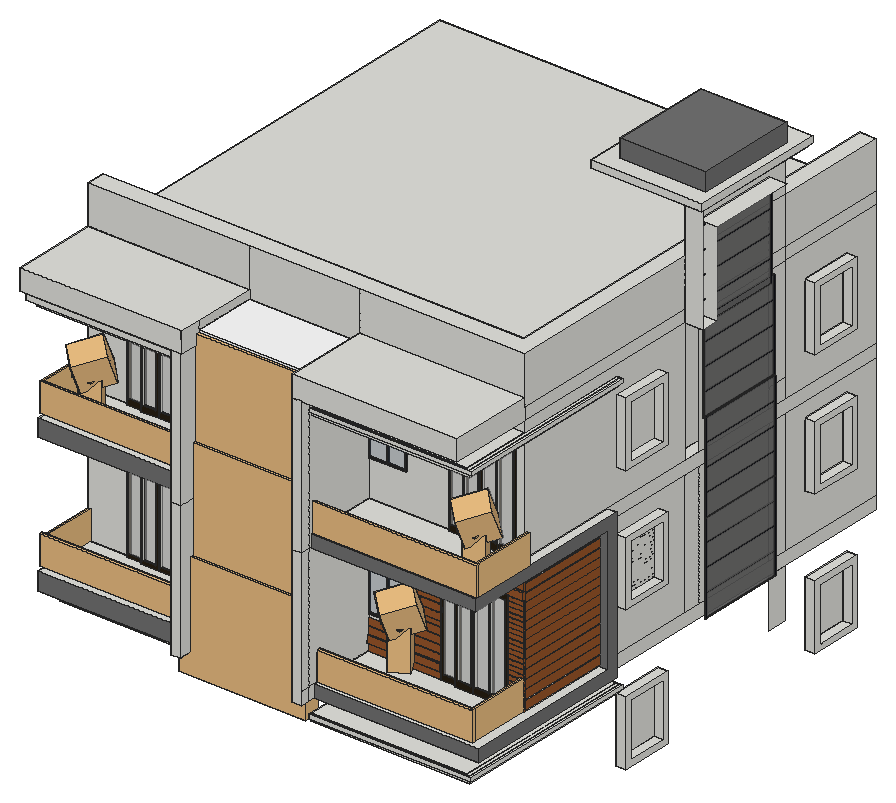
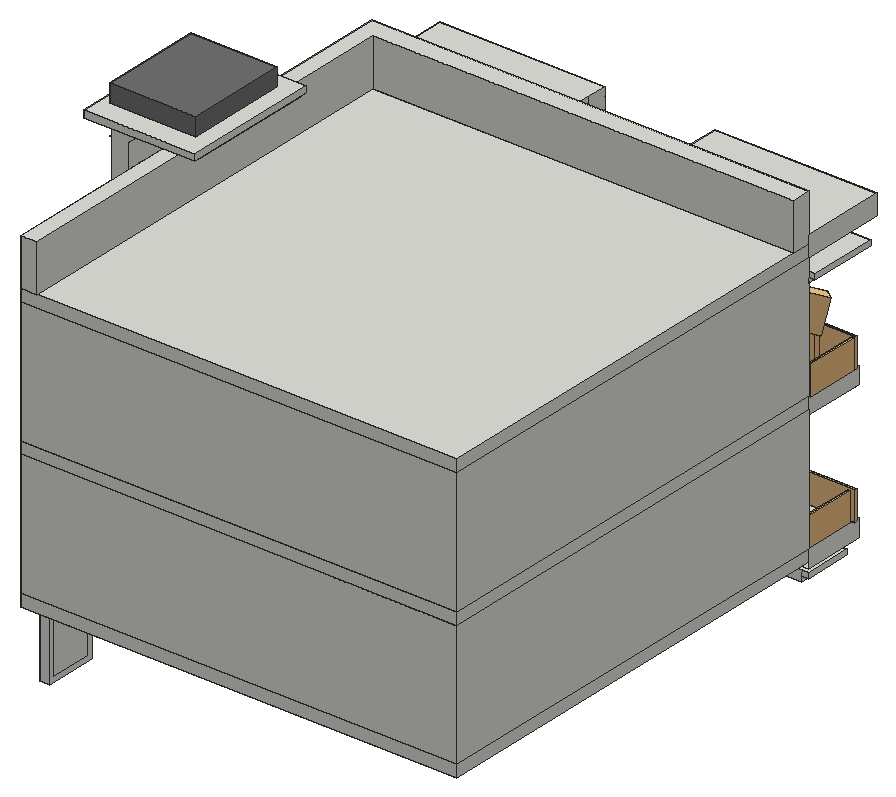
# SketchUp Ruby script. Lengths in inches.
U = 1.inch
M = Sketchup.active_model
def pt(a) = Geom::Point3d.new(a.map { |v| v * U })
def face(e, loops, mat)
  f = e.add_face(loops[0].map { |a| pt(a) })
  loops[1..].each { |l| e.add_face(l.map { |a| pt(a) }).erase! }
  f.material = f.back_material = mat if mat
  f
end
# faces: each face lists its corners as indices into pts; further lists are holes
def faces(e, pts, list, mat = nil) = list.each { |f| face(e, (f[0].is_a?(Array) ? f : [f]).map { |l| l.map { |i| pts[i] } }, mat) }
# xy, xz, yz: faces in a plane at the given z, y or x. An outline is a flat list of corners, or four numbers for a rectangle; further outlines are holes
def ring(l) = l.size == 4 ? [[l[0], l[1]], [l[2], l[1]], [l[2], l[3]], [l[0], l[3]]] : l.each_slice(2).to_a
def flat(e, list, mat, &to3) = list.each { |f| face(e, (f[0].is_a?(Array) ? f : [f]).map { |l| ring(l).map { |u, v| to3.(u, v) } }, mat) }
def xy(e, z, list, mat = nil) = flat(e, list, mat) { |x, y| [x, y, z] }
def xz(e, y, list, mat = nil) = flat(e, list, mat) { |x, z| [x, y, z] }
def yz(e, x, list, mat = nil) = flat(e, list, mat) { |y, z| [x, y, z] }
def lines(e, pts, list) = list.each { |a, b| e.add_line(pt(pts[a]), pt(pts[b])) }
# prism: a flat outline (further loops are holes) pulled along v
def prism(e, loops, v, mat = nil)
  f = face(e, loops, mat); d = Geom::Vector3d.new(v.map { |x| x * U })
  f.pushpull(f.normal.samedirection?(d) ? d.length : -d.length)
end
def box(e, o, s, mat = nil) = prism(e, [[o, [o[0] + s[0], o[1], o[2]], [o[0] + s[0], o[1] + s[1], o[2]], [o[0], o[1] + s[1], o[2]]]], [0, 0, s[2]], mat)
def at(x, y, z, deg = 0) = Geom::Transformation.translation(pt([x, y, z])) * Geom::Transformation.rotation(ORIGIN, Z_AXIS, deg.degrees)
def axes(o, x, y, z) = Geom::Transformation.new([*x, 0, *y, 0, *z, 0, *pt(o).to_a, 1])
def part(name) = M.definitions.add(name)
# library, detail: a bought-in or finely detailed component or shape, given as its bounding box
def library(name, o, s) = part(name).tap { |d| box(d.entities, o, s) }
def detail(e, o, s) = box(e.add_group.entities, o, s)
def put(e, d, t, mat = nil) = e.add_instance(d, t).tap { |i| i.material = mat if mat }
def group(e, t, mat = nil) = e.add_group.tap { |g| g.transformation = t; g.material = mat if mat }.entities
root = M.entities
M.materials.add("Material__1").color = [51, 42, 44]
M.materials.add("Material__2").color = [97, 132, 37]
M.materials.add("[0136_Charcoal]").color = [35, 35, 35]
M.materials.add("[Color M00]").color = [255, 255, 255]
M.materials.add("[Color M05]").color = [114, 114, 114]
M.materials.add("[Translucent Glass Gray]2").color = [201, 201, 201]
M.materials["[Translucent Glass Gray]2"].alpha = 0.5
M.materials.add("[Translucent_Glass_Blue]").color = [68, 104, 165]
M.materials["[Translucent_Glass_Blue]"].alpha = 0.07
M.materials.add("[Translucent_Glass_Green_Dark]").color = [33, 68, 103]
M.materials["[Translucent_Glass_Green_Dark]"].alpha = 0.08
M.materials.add("[Wood Cherry Original]").color = [152, 86, 42]
M.materials.add("oak swatch").color = [40, 31, 19]
M.materials.add("{045efeae-c101-a24d-bd9b-6f5600100adb}").color = [102, 102, 102]
M.materials["{045efeae-c101-a24d-bd9b-6f5600100adb}"].alpha = 0.7
M.materials.add("{16756a1b-d383-d94f-ad82-104813d2624f}").color = [19, 21, 27]
c1 = part("Group\#20")
xy(c1.entities,0,[[[0,0,50.8125,62.9375],[5.49,5.49,45.32,57.45]],[5.49,5.49,45.32,57.45]])
xy(c1.entities,9.5625,[[[0,0,50.8125,62.9375],[5.49,5.49,45.32,57.45]]])
xz(c1.entities,0,[[0,0,50.8125,9.5625]])
xz(c1.entities,5.49,[[5.49,0,45.32,9.5625]])
xz(c1.entities,57.45,[[5.49,0,45.32,9.5625]])
xz(c1.entities,62.9375,[[0,0,50.8125,9.5625]])
yz(c1.entities,0,[[0,0,62.9375,9.5625]])
yz(c1.entities,5.49,[[5.49,0,57.45,9.5625]])
yz(c1.entities,45.32,[[5.49,0,57.45,9.5625]])
yz(c1.entities,50.8125,[[0,0,62.9375,9.5625]])
c2 = library("Facade Louver",[-2.17,-1,-2.17],[122.45,14.39,102.76])
c3 = part("Group\#29")
xy(c3.entities,-4.5625,[[0,-81.875,145.875,0]])
xy(c3.entities,0.59,[[-6.375,-89.375,-6.375,0,0,0,0,-81.875,145.875,-81.875,145.875,-89.375]])
xy(c3.entities,5.73,[[-6.375,-89.375,145.875,0]])
xz(c3.entities,-89.375,[[-6.375,0.59,145.875,5.73]])
xz(c3.entities,-81.875,[[0,-4.5625,145.875,0.59]])
xz(c3.entities,0,[[0,-4.5625,145.875,5.73],[-6.375,0.59,0,5.73]])
yz(c3.entities,-6.375,[[-89.375,0.59,0,5.73]])
yz(c3.entities,0,[[-81.875,-4.5625,0,0.59]])
yz(c3.entities,145.875,[[-81.875,-4.5625,0,-4.5625,0,5.73,-89.375,5.73,-89.375,0.59,-81.875,0.59]])
c4 = part("Furniture_0DcpanrIvuI8n_9Ae92L5A")
g1 = group(c4.entities,at(0,0,0))
box(g1,[-19.29,-0.2,0.39],[38.58,0.4,83.86],"{045efeae-c101-a24d-bd9b-6f5600100adb}")
g2 = group(c4.entities,at(0,0,0))
box(g2,[-19.68,-0.59,63.39],[39.36,1.18,0.39],"{16756a1b-d383-d94f-ad82-104813d2624f}")
box(g2,[-19.68,-0.59,42.52],[39.36,1.18,0.39],"{16756a1b-d383-d94f-ad82-104813d2624f}")
box(g2,[-19.68,-0.59,21.26],[39.36,1.18,0.39],"{16756a1b-d383-d94f-ad82-104813d2624f}")
xy(g2,0,[[-19.68,-0.59,19.68,0.59]],"{16756a1b-d383-d94f-ad82-104813d2624f}")
xy(g2,0.39,[[-19.68,-0.59,-19.29,0.59],[-19.68,-0.59,19.68,0.59],[19.29,-0.59,19.68,0.59]],"{16756a1b-d383-d94f-ad82-104813d2624f}")
xy(g2,84.25,[[-19.68,-0.59,19.68,0.59]],"{16756a1b-d383-d94f-ad82-104813d2624f}")
xy(g2,84.65,[[-19.68,-0.59,-19.29,0.59],[-19.68,-0.59,19.68,0.59],[19.29,-0.59,19.68,0.59]],"{16756a1b-d383-d94f-ad82-104813d2624f}")
xz(g2,-0.59,[[-19.68,0,19.68,0.39],[-19.68,0.39,-19.29,84.65],[19.29,0.39,19.68,84.65],[-19.68,84.25,19.68,84.65]],"{16756a1b-d383-d94f-ad82-104813d2624f}")
xz(g2,0.59,[[-19.68,0,19.68,0.39],[-19.68,0.39,-19.29,84.65],[19.29,0.39,19.68,84.65],[-19.68,84.25,19.68,84.65]],"{16756a1b-d383-d94f-ad82-104813d2624f}")
yz(g2,-19.68,[[-0.59,0,0.59,0.39],[-0.59,0.39,0.59,84.65],[-0.59,84.25,0.59,84.65]],"{16756a1b-d383-d94f-ad82-104813d2624f}")
yz(g2,-19.29,[[-0.59,0.39,0.59,84.65]],"{16756a1b-d383-d94f-ad82-104813d2624f}")
yz(g2,19.29,[[-0.59,0.39,0.59,84.65]],"{16756a1b-d383-d94f-ad82-104813d2624f}")
yz(g2,19.68,[[-0.59,0,0.59,0.39],[-0.59,0.39,0.59,84.65],[-0.59,84.25,0.59,84.65]],"{16756a1b-d383-d94f-ad82-104813d2624f}")
c5 = part("Glass Window")
put(c5.entities,c4,at(0,0,-42.32))
c6 = part("Group\#7")
box(c6.entities,[0,0,0],[1.77,4.72,80.31],"oak swatch")
c7 = part("Exterior Sliding Doors")
xy(c7.entities,0,[[1.77,33.07,3.54,70.87],[1.77,70.87,3.54,108.66]])
xy(c7.entities,0,[[0,0,1.77,33.07],[0,108.66,1.77,141.73]],"oak swatch")
xy(c7.entities,4.72,[[0,4.72,1.77,33.07],[1.77,37.8,3.54,66.14],[1.77,75.88,3.54,103.9375],[0,108.66,1.77,137.01]],"oak swatch")
xy(c7.entities,75.59,[[1.77,37.8,3.54,66.14],[1.77,75.88,3.54,103.9375]])
xy(c7.entities,75.59,[[0,4.72,1.77,33.07],[0,108.66,1.77,137.01]],"oak swatch")
xy(c7.entities,80.31,[[0,0,1.77,33.07],[1.77,33.07,3.54,70.87],[1.77,70.87,3.54,108.66],[0,108.66,1.77,141.73]],"oak swatch")
xz(c7.entities,0,[[0,0,1.77,80.31]],"oak swatch")
xz(c7.entities,4.72,[[0,4.72,1.77,75.59]],"oak swatch")
xz(c7.entities,33.07,[[0,0,1.77,4.72],[1.77,0,3.54,80.31],[0,75.59,1.77,80.31]],"oak swatch")
xz(c7.entities,37.8,[[1.77,4.72,3.54,75.59]])
xz(c7.entities,66.14,[[1.77,4.72,3.54,75.59]],"oak swatch")
xz(c7.entities,70.87,[[1.77,0,3.54,80.31]])
xz(c7.entities,75.88,[[1.77,4.72,3.54,75.59]])
xz(c7.entities,103.9375,[[1.77,4.72,3.54,75.59]],"oak swatch")
xz(c7.entities,108.66,[[1.77,4.72,3.54,75.59]])
xz(c7.entities,108.66,[[0,0,3.54,4.72],[0,75.59,3.54,80.31]],"oak swatch")
xz(c7.entities,137.01,[[0,4.72,1.77,75.59]],"oak swatch")
xz(c7.entities,141.73,[[0,0,1.77,80.31]],"oak swatch")
yz(c7.entities,0,[[0,0,33.07,0,33.07,4.72,4.72,4.72,4.72,75.59,33.07,75.59,33.07,80.31,0,80.31],[108.66,0,141.73,0,141.73,80.31,108.66,80.31,108.66,75.59,137.01,75.59,137.01,4.72,108.66,4.72]],"oak swatch")
yz(c7.entities,1.77,[[4.72,4.72,33.07,75.59],[37.8,4.72,66.14,75.59],[75.88,4.72,103.9375,75.59],[108.66,4.72,137.01,75.59]],"[Translucent Glass Gray]2")
yz(c7.entities,1.77,[[0,0,33.07,0,33.07,4.72,4.72,4.72,4.72,75.59,33.07,75.59,33.07,80.31,0,80.31],[[33.07,0,70.87,80.31],[37.8,4.72,66.14,75.59]],[[70.87,0,141.73,80.31],[108.66,4.72,137.01,75.59],[75.88,4.72,103.9375,75.59]]],"oak swatch")
yz(c7.entities,3.54,[[[33.07,0,70.87,80.31],[37.8,4.72,66.14,75.59]],[[70.87,0,108.66,80.31],[75.88,4.72,103.9375,75.59]]],"oak swatch")
put(c7.entities,c6,at(0,33.07,0))
put(c7.entities,c6,at(0,103.9375,0))
c8 = part("Group\#15")
box(c8.entities,[0,0,0],[15.2,4.13,1.25])
c9 = library("Glass Railings(black Handrails)",[-57.04,-132.55,0],[169.29,2.52,28.17])
c10 = part("Group\#13")
box(c10.entities,[0,-0.9375,0],[71.3,0.9375,6.72])
c11 = part("Group\#8")
box(c11.entities,[61.69,-1.625,-2],[88.94,1.625,7.49])
c12 = library("\#1",[-138.85,-135.75,0],[277.7,270.97,9.64])
c13 = library("\#2",[-34.84,-73.35,-33.91],[69.68,146.26,68.31])
c14 = library("\#5",[-4127.85,-1300.75,-2324.72],[5349.84,4521.24,5423.31])
c15 = part("\#3")
put(c15.entities,c14,at(450.18,-1111.4375,0),"Material__2")
c16 = part("12")
put(c16.entities,c12,axes([-49.79,-36.9375,349.64],[0.59279,0,0],[0,0.59279,0],[0,0,0.59279]),"Material__1")
put(c16.entities,c13,axes([-39.24,-18.18,177.19],[1.20819,-2.09264,0],[0,0,2.41638],[2.09264,1.20819,0]))
put(c16.entities,c15,axes([-83.44,-46.04,442.44],[-0.03636,-0.03293,-0.01473],[-0.00083,-0.02391,0.05549],[0.02997,-0.02791,-0.01158]))
c17 = part("Group\#14")
box(c17.entities,[0,0,0],[34.99,6.92,0.9375])
c18 = part("Two-panel window \#1")
xy(c18.entities,-18,[[0,-31,2,35]],"[0136_Charcoal]")
xy(c18.entities,-16,[[0,-29,0.9375,33],[0.9375,-29,1.125,33],[1.125,-29,2,1],[1.125,3,2,33]],"[0136_Charcoal]")
xy(c18.entities,76,[[0,-29,0.9375,33],[0.9375,-29,1.125,33],[1.125,-29,2,1],[1.125,3,2,33]],"[0136_Charcoal]")
xy(c18.entities,78,[[0,-31,2,35]],"[0136_Charcoal]")
xz(c18.entities,-31,[[0,-18,2,78]],"[0136_Charcoal]")
xz(c18.entities,-29,[[0,-16,0.9375,76],[0.9375,-16,1.125,76],[1.125,-16,2,76]],"[0136_Charcoal]")
xz(c18.entities,1,[[1.125,-16,2,76]],"[0136_Charcoal]")
xz(c18.entities,3,[[1.125,-16,2,76]],"[0136_Charcoal]")
xz(c18.entities,33,[[0,-16,0.9375,76],[0.9375,-16,1.125,76],[1.125,-16,2,76]],"[0136_Charcoal]")
xz(c18.entities,35,[[0,-18,2,78]],"[0136_Charcoal]")
yz(c18.entities,0,[[[-31,-18,35,78],[-29,-16,33,76]]],"[0136_Charcoal]")
yz(c18.entities,0.9375,[[-29,-16,33,76]],"[Translucent_Glass_Blue]")
yz(c18.entities,1.125,[[1,-16,3,76]],"[0136_Charcoal]")
yz(c18.entities,1.125,[[-29,-16,1,76],[3,-16,33,76]],"[Translucent_Glass_Green_Dark]")
yz(c18.entities,2,[[[-31,-18,35,78],[-29,-16,1,76],[3,-16,33,76]]],"[0136_Charcoal]")
c19 = part("Two-panel window")
put(c19.entities,c18,axes([-31.84,50.72,0],[1,0,0],[0,1.1,0],[0,0,1]))
c20 = part("normal window")
put(c20.entities,c19,axes([114.26,44.3125,18],[0,1,0],[-0.90909,0,0],[0,0,1]))
prism(root,[[[317.76,103.01,369.07],[468.38,103.01,369.07],[468.38,173.57,369.07],[468.38,283.99,369.07],[474.57,283.99,369.07],[474.57,100.51,369.07],[317.76,100.51,369.07],[317.76,100.69,369.07]]],[0,0,3.5])
xy(root,378.5,[[45.88,113.44,191.76,173.57]])
xy(root,384,[[317.76,107.01,317.76,173.57,468.38,173.57,468.38,273.38,477.41,273.38,477.41,107.01]])
xy(root,396,[[317.76,107.01,477.41,107.01,477.41,262.5,468.38,262.5,468.38,173.57,317.76,173.57],[200.76,112.2,308.76,121.2],[45.88,113.44,191.76,173.57],[200.76,121.2,308.76,121.2,308.76,182.57,425.76,182.57,425.76,442.69,83.76,442.69,83.76,182.57,200.76,182.57],[45.88,173.57,200.76,173.57,200.76,182.57,83.76,182.57,83.76,442.69,425.76,442.69,425.76,182.57,308.76,182.57,308.76,173.57,468.38,173.57,468.38,598.82,45.88,598.82]])
xy(root,500.875,[[202.09,121.2,202.09,173.57,200.76,173.57,200.76,182.57,56.45,182.57,56.45,442.69,456.2,442.69,456.2,182.57,308.76,182.57,308.76,121.2]])
xy(root,511.75,[[45.88,113.44,191.76,173.57]])
xy(root,516,[[308.76,91.69,317.76,173.57],[200.76,112.2,308.76,121.2],[317.76,113.44,468.38,173.57],[45.88,173.57,200.76,173.57,200.76,182.57,83.76,182.57,83.76,442.69,425.76,442.69,425.76,182.57,308.76,182.57,308.76,173.57,468.38,173.57,468.38,598.82,45.88,598.82]])
xy(root,516.15,[[317.76,102.75,317.76,113.44,468.38,113.44,468.38,262.5,477.41,262.5,477.41,102.75]])
xy(root,528,[[317.76,102.75,477.41,102.75,477.41,273.38,468.38,273.38,468.38,113.44,317.76,113.44],[200.76,112.2,308.76,121.2],[45.88,113.44,191.76,173.57],[317.76,113.44,468.38,173.57],[200.76,121.2,308.76,121.2,308.76,182.57,456.2,182.57,456.2,442.69,56.45,442.69,56.45,182.57,200.76,182.57],
  [45.88,173.57,200.76,173.57,200.76,182.57,56.45,182.57,56.45,442.69,456.2,442.69,456.2,182.57,308.76,182.57,308.76,173.57,468.38,173.57,468.38,598.82,45.88,598.82]])
xy(root,634.26,[[317.76,101.26,317.76,103.01,468.38,103.01,468.38,284.44,475.01,284.44,475.01,101.26]])
xy(root,637.76,[[317.76,101.26,475.01,101.26,475.01,284.44,468.38,284.44,468.38,103.01,317.76,103.01]])
xy(root,648,[[45.88,91.69,83.76,173.57],[83.76,91.69,191.76,173.57],[191.76,91.69,200.76,173.57],[200.76,91.69,202.09,112.2],[308.76,91.69,317.76,173.57],
  [317.76,91.69,425.76,173.57],[425.76,91.69,468.38,173.57],[200.76,112.2,202.09,121.2],[202.09,112.2,308.76,121.2],[200.76,121.2,202.09,173.57],
  [45.88,173.57,200.76,173.57,200.76,182.57,56.45,182.57,56.45,442.69,456.2,442.69,456.2,182.57,308.76,182.57,308.76,173.57,468.38,173.57,468.38,598.82,45.88,598.82],[468.38,367.14,485.45,384.58]])
xy(root,660,[[45.88,173.57,45.88,192.04,452.39,192.04,452.39,598.82,468.38,598.82,468.38,173.57]])
xy(root,660,[[202.09,112.2,308.76,173.57]],"[Color M00]")
xy(root,668.0625,[[45.88,91.69,202.09,173.57],[308.76,91.69,468.38,173.57]])
xy(root,705.6875,[[45.88,173.57,468.38,173.57,468.38,598.82,452.39,598.82,452.39,192.04,45.88,192.04]])
xy(root,729.3125,[[468.38,384.58,485.45,469.33]])
xy(root,754.625,[[382.24,360.76,485.45,367.14],[485.45,360.76,489.76,488.7],[382.24,367.14,468.38,488.7],[468.38,367.14,485.45,488.7],[382.24,488.7,489.76,495.14]])
xy(root,761.4375,[[[382.24,360.76,489.76,495.14],[398.09,376.66,481.09,474.6]]])
xy(root,778.875,[[398.09,376.66,481.09,474.6]],"[Color M05]")
xz(root,91.69,[[191.76,383.9375,200.76,384],[191.76,384,200.76,516],[308.76,384,317.76,516],[191.76,516,200.76,648],[308.76,516,317.76,648],
  [45.88,648,202.09,668.0625],[308.76,648,468.38,668.0625]])
xz(root,101.26,[[317.76,634.26,475.01,637.76]])
xz(root,102.75,[[317.76,516.15,477.41,528]],"[Color M05]")
xz(root,103.01,[[317.76,634.26,468.38,637.76]])
xz(root,107.01,[[317.76,384,477.41,396]],"[Color M05]")
xz(root,112.2,[[200.76,384,308.76,396],[200.76,396,308.76,516],[200.76,516,308.76,528],[200.76,528,308.76,648]])
xz(root,112.2,[[202.09,648,308.76,660]],"[Color M00]")
xz(root,113.44,[[317.76,516,468.38,516.15],[317.76,516.15,468.38,528]])
xz(root,113.44,[[45.88,378.5,191.76,396],[45.88,511.75,191.76,528]],"[Color M05]")
xz(root,121.2,[[200.76,396,200.76,516,202.09,516,202.09,500.875,308.76,500.875,308.76,396],[202.09,500.875,308.76,516],[202.09,516,308.76,528],[200.76,528,202.09,648],[202.09,528,308.76,648]])
xz(root,173.57,[[191.76,383.9375,200.76,396],[308.76,384,317.76,396],[45.88,396,191.76,511.75],[389.06,396,468.38,396,468.38,508.52,317.76,508.52,317.76,402.72,389.06,402.72],[200.76,500.875,202.09,648],
  [45.88,511.75,191.76,516],[191.76,516,200.76,528],[308.76,516,317.76,528],[317.76,516,468.38,528],[45.88,528,191.76,630.49],
  [317.76,528,468.38,648],[45.88,641.6,191.76,648],[45.88,648,202.09,660],[308.76,648,468.38,660],[45.88,660,202.09,668.0625],
  [202.09,660,308.76,705.6875],[308.76,660,468.38,668.0625],[45.88,668.0625,202.09,705.6875],[308.76,668.0625,468.38,705.6875]])
xz(root,182.57,[[83.76,396,200.76,500.875],[308.76,396,425.76,500.875],[56.45,500.875,83.76,500.875,83.76,516,200.76,516,200.76,528,56.45,528],[83.76,500.875,200.76,516],[308.76,500.875,425.76,516],
  [425.76,500.875,456.2,500.875,456.2,528,308.76,528,308.76,516,425.76,516],[56.45,528,200.76,648],[308.76,528,456.2,648]])
xz(root,192.04,[[45.88,660,452.39,705.6875]])
xz(root,262.5,[[468.38,396,477.41,516.15]],"[Color M05]")
xz(root,273.38,[[468.38,384,477.41,528]])
xz(root,284.44,[[468.38,634.26,475.01,637.76]])
xz(root,360.76,[[382.24,754.625,489.76,761.4375]])
xz(root,367.14,[[468.38,648,485.45,754.625]])
xz(root,376.66,[[398.09,761.4375,481.09,778.875]],"[Color M05]")
xz(root,384.58,[[468.38,648,485.45,729.3125]])
xz(root,442.69,[[83.76,396,425.76,500.875],[56.45,500.875,56.45,528,456.2,528,456.2,500.875,425.76,500.875,425.76,516,83.76,516,83.76,500.875],[83.76,500.875,425.76,516],[56.45,528,456.2,648]])
xz(root,474.6,[[398.09,761.4375,481.09,778.875]],"[Color M05]")
xz(root,495.14,[[382.24,754.625,489.76,761.4375]])
xz(root,598.82,[[45.88,396,468.38,516],[45.88,528,468.38,648],[452.39,660,468.38,705.6875]])
yz(root,45.88,[[113.44,378.5,173.57,396],[173.57,396,598.82,516],[113.44,511.75,173.57,528],[173.57,528,598.82,648],[91.69,648,173.57,668.0625],
  [173.57,660,192.04,705.6875]])
yz(root,56.45,[[182.57,500.875,442.69,528],[182.57,528,442.69,648]])
yz(root,83.76,[[182.57,396,442.69,516]])
yz(root,191.76,[[113.44,378.5,173.57,396],[91.69,383.9375,100.69,384],[91.69,384,100.69,516],[113.44,511.75,173.57,528],[91.69,516,91.69,648,100.69,648,100.69,528,113.44,528,113.44,516],
  [100.69,528,173.57,648]])
yz(root,200.76,[[91.69,383.9375,112.2,384],[112.2,383.9375,121.2,396],[121.2,383.9375,173.57,384],[91.69,384,112.2,516],[121.2,384,173.57,396],
  [112.2,396,121.2,516],[121.2,396,182.57,396,182.57,500.875,173.57,500.875,173.57,516,121.2,516],[173.57,500.875,182.57,516],[91.69,516,112.2,648],[112.2,516,121.2,528],
  [121.2,516,173.57,528],[173.57,516,182.57,528],[121.2,528,173.57,648],[173.57,528,182.57,648],[91.69,659.75,92.36,660]])
yz(root,202.09,[[121.2,500.875,173.57,648],[91.69,648,112.2,668.0625],[112.2,648,173.57,660],[112.2,660,173.57,668.0625]])
yz(root,308.76,[[91.69,384,112.2,516],[112.2,384,121.2,396],[121.2,384,173.57,396],[121.2,396,182.57,500.875],[121.2,500.875,173.57,516],
  [173.57,500.875,182.57,516],[91.69,516,112.2,648],[112.2,516,121.2,528],[121.2,516,173.57,528],[173.57,516,182.57,528],
  [121.2,528,173.57,648],[173.57,528,182.57,648],[91.69,648,112.2,668.0625],[112.2,648,173.57,660],[112.2,660,173.57,668.0625]])
yz(root,317.76,[[91.69,384,100.69,396],[91.69,384,100.69,396],[100.69,384,107.01,396],[107.01,384,173.57,396],[91.69,396,100.69,516],
  [100.69,396,173.57,516],[91.69,516,100.69,648],[100.69,516,113.44,516,113.44,516.15,102.75,516.15,102.75,528,173.57,528,173.57,648,100.69,648],[113.44,516,173.57,528],[101.26,634.26,103.01,637.76]])
yz(root,382.24,[[360.76,754.625,495.14,761.4375]])
yz(root,398.09,[[376.66,761.4375,474.6,778.875]],"[Color M05]")
yz(root,425.76,[[182.57,396,442.69,516]])
yz(root,452.39,[[192.04,660,598.82,705.6875]])
yz(root,456.2,[[182.57,500.875,442.69,528],[182.57,528,442.69,648]])
yz(root,468.38,[[469.33,335.6875,488.7,384],[173.57,384,273.38,396],[367.14,384,384.58,396],[469.33,384,488.7,396],[173.57,396,262.5,516],
  [262.5,396,273.38,516],[273.38,396,367.14,516],[367.14,396,384.58,516],[384.58,396,469.33,516],[469.33,396,488.7,516],
  [488.7,396,598.82,516],[113.44,516,173.57,516.15],[262.5,516,262.5,516.15,173.57,516.15,173.57,528,273.38,528,273.38,516],[367.14,516,384.58,528],[469.33,516,488.7,528],
  [113.44,516.15,173.57,528],[173.57,528,367.14,528,367.14,648,173.57,648,173.57,637.76,284.44,637.76,284.44,634.26,173.57,634.26],[384.58,528,469.33,648],[469.33,528,488.7,546.9375],[488.7,528,598.82,648],
  [469.33,546.9375,488.7,648],[103.01,634.26,173.57,637.76],[173.57,634.26,284.44,637.76],[91.69,648,173.57,668.0625],[367.14,648,384.58,660],
  [384.58,648,469.33,660],[469.33,648,488.7,660],[173.57,660,367.14,705.6875],[367.14,660,384.58,705.6875],[384.58,660,469.33,705.6875],
  [469.33,660,488.7,705.6875],[488.7,660,598.82,705.6875],[367.14,705.6875,367.14,754.625,488.7,754.625,488.7,705.6875,469.33,705.6875,469.33,729.3125,384.58,729.3125,384.58,705.6875],[384.58,705.6875,469.33,729.3125]])
yz(root,475.01,[[101.26,634.26,284.44,637.76]])
yz(root,477.41,[[107.01,384,273.38,384,273.38,528,102.75,528,102.75,516.15,262.5,516.15,262.5,396,107.01,396]],"[Color M05]")
yz(root,481.09,[[376.66,761.4375,474.6,778.875]],"[Color M05]")
yz(root,489.76,[[360.76,754.625,495.14,761.4375]])
p = [[308.59,91.69,395.75],[308.59,91.69,396],[308.59,91.69,527.75],[308.59,91.69,528],[200.76,112.2,659.75],[200.76,112.2,660],
  [308.59,91.69,659.75],[308.59,91.69,660],[200.76,91.69,660],[200.76,91.69,668.0625]]
lines(root,p,[[0,1],[2,3],[4,5],[6,7],[8,9]])
put(root,c1,axes([468.38,283.99,300.58],[0,1,0],[0,0,1],[1,0,0]))
put(root,c1,axes([468.38,512.67,300.58],[0,1,0],[0,0,1],[1,0,0]))
put(root,c2,at(192.27,104.35,366.41))
put(root,c3,axes([52.26,173.57,369.17],[1,0,0],[0,0.52,0],[0,0,1]))
g3 = group(root,at(317.76,173.57,365.57))
box(g3,[0,-70.5625,0],[154.0625,180.75,7.01])
g4 = group(root,at(74.76,451.69,384))
box(g4,[-28.875,-278.125,0],[422.5,425.25,12])
put(root,c5,axes([474.13,426.95,429.12],[0,-2.15265,0],[1,0,0],[0,0,1.03]))
put(root,c7,axes([84.67,173.57,393.25],[0,-1,0],[0.4524,0,0],[0,0,1.21]))
put(root,c8,axes([453.18,173.57,395.46],[1,0,0],[0,0,1],[0,-1,0]),"[Wood Cherry Original]")
put(root,c9,axes([-84.15,140.24,395.92],[0,0.29695,0],[-1,0,0],[0,0,1]))
put(root,c9,axes([368.53,243.48,396],[0.89,0,0],[0,1,0],[0,0,1]))
put(root,c7,axes([389.06,173.57,396],[0,-1,0],[0.4524,0,0],[0,0,1.21]))
put(root,c10,at(317.76,173.57,396),"[Wood Cherry Original]")
put(root,c9,axes([335.83,132.73,396.48],[0,0.36382,0],[-1,0,0],[0,0,1]))
put(root,c9,axes([93.65,251.23,396.6875],[0.89,0,0],[0,1,0],[0,0,1]))
put(root,c11,at(467.95,111.88,400.08,90),"[Wood Cherry Original]")
put(root,c8,axes([453.18,173.57,400.33],[1,0,0],[0,0,1],[0,-1,0]),"[Wood Cherry Original]")
put(root,c10,at(317.76,171.32,404),"[Wood Cherry Original]")
put(root,c8,axes([453.18,173.57,404.96],[1,0,0],[0,0,1],[0,-1,0]),"[Wood Cherry Original]")
put(root,c11,at(467.95,111.88,409.39,90),"[Wood Cherry Original]")
put(root,c8,axes([453.18,173.57,409.65],[1,0,0],[0,0,1],[0,-1,0]),"[Wood Cherry Original]")
put(root,c10,at(317.76,173.57,410.9),"[Wood Cherry Original]")
put(root,c8,axes([453.18,173.57,414.21],[1,0,0],[0,0,1],[0,-1,0]),"[Wood Cherry Original]")
put(root,c11,at(467.95,111.88,418.26,90),"[Wood Cherry Original]")
put(root,c10,at(317.76,173.57,418.4),"[Wood Cherry Original]")
put(root,c8,axes([453.18,173.57,418.9],[1,0,0],[0,0,1],[0,-1,0]),"[Wood Cherry Original]")
put(root,c16,axes([382.94,137.37,419.89],[0.1092,0,0],[0,0.1092,0],[0,0,0.1092]))
put(root,c8,axes([453.18,173.57,423.52],[1,0,0],[0,0,1],[0,-1,0]),"[Wood Cherry Original]")
put(root,c11,at(467.95,111.88,426.95,90),"[Wood Cherry Original]")
put(root,c17,axes([354.07,173.57,426.05],[1,0,0],[0,0,1],[0,-1,0]),"[Wood Cherry Original]")
put(root,c8,axes([453.18,173.57,428.08],[1,0,0],[0,0,1],[0,-1,0]),"[Wood Cherry Original]")
put(root,c20,axes([299.72,167.1875,428.35],[0.5481,0,0],[0,0.441,0],[0,0,0.63]))
put(root,c8,axes([453.18,173.57,432.77],[1,0,0],[0,0,1],[0,-1,0]),"[Wood Cherry Original]")
put(root,c11,at(467.95,111.88,435.64,90),"[Wood Cherry Original]")
put(root,c17,axes([354.07,173.57,433.86],[1,0,0],[0,0,1],[0,-1,0]),"[Wood Cherry Original]")
put(root,c8,axes([453.18,173.57,437.4],[1,0,0],[0,0,1],[0,-1,0]),"[Wood Cherry Original]")
put(root,c1,axes([468.38,283.99,438.64],[0,1,0],[0,0,1],[1,0,0]))
put(root,c1,axes([468.38,512.67,438.64],[0,1,0],[0,0,1],[1,0,0]))
g5 = group(root,at(354.07,173.57,441.54),"[Wood Cherry Original]")
box(g5,[0,-0.9375,0],[34.99,0.9375,4.26])
put(root,c8,axes([453.18,173.57,441.83],[1,0,0],[0,0,1],[0,-1,0]),"[Wood Cherry Original]")
put(root,c11,at(467.95,111.88,444.26,90),"[Wood Cherry Original]")
put(root,c8,axes([453.18,173.57,446.46],[1,0,0],[0,0,1],[0,-1,0]),"[Wood Cherry Original]")
put(root,c17,axes([354.07,173.57,446.49],[1,0,0],[0,0,1],[0,-1,0]),"[Wood Cherry Original]")
put(root,c11,at(467.95,111.88,452.45,90),"[Wood Cherry Original]")
put(root,c8,axes([453.18,173.57,451.08],[1,0,0],[0,0,1],[0,-1,0]),"[Wood Cherry Original]")
put(root,c17,axes([354.19,173.57,453.99],[1,0,0],[0,0,1],[0,-1,0]),"[Wood Cherry Original]")
put(root,c8,axes([453.18,173.57,455.71],[1,0,0],[0,0,1],[0,-1,0]),"[Wood Cherry Original]")
put(root,c11,at(467.95,111.88,460.64,90),"[Wood Cherry Original]")
put(root,c8,axes([453.18,173.57,460.21],[1,0,0],[0,0,1],[0,-1,0]),"[Wood Cherry Original]")
put(root,c17,axes([354.07,173.625,461.83],[1,0,0],[0,0,1],[0,-1,0]),"[Wood Cherry Original]")
put(root,c2,at(194.8,107.3,464.04))
put(root,c8,axes([453.18,173.57,464.71],[1,0,0],[0,0,1],[0,-1,0]),"[Wood Cherry Original]")
put(root,c11,at(467.95,111.88,468.7,90),"[Wood Cherry Original]")
put(root,c8,axes([453.18,173.57,469.21],[1,0,0],[0,0,1],[0,-1,0]),"[Wood Cherry Original]")
put(root,c17,axes([354.07,173.625,469.39],[1,0,0],[0,0,1],[0,-1,0]),"[Wood Cherry Original]")
put(root,c5,axes([474.13,426.95,515.89],[0,-2.15265,0],[1,0,0],[0,0,1.03]))
put(root,c8,axes([453.18,173.57,473.71],[1,0,0],[0,0,1],[0,-1,0]),"[Wood Cherry Original]")
put(root,c11,at(467.95,111.88,476.76,90),"[Wood Cherry Original]")
put(root,c17,axes([354.07,173.625,476.83],[1,0,0],[0,0,1],[0,-1,0]),"[Wood Cherry Original]")
put(root,c8,axes([453.18,173.57,478.4],[1,0,0],[0,0,1],[0,-1,0]),"[Wood Cherry Original]")
put(root,c11,at(467.95,111.88,484.76,90),"[Wood Cherry Original]")
put(root,c8,axes([453.18,173.57,482.96],[1,0,0],[0,0,1],[0,-1,0]),"[Wood Cherry Original]")
put(root,c17,axes([354.07,173.625,484.22],[1,0,0],[0,0,1],[0,-1,0]),"[Wood Cherry Original]")
put(root,c8,axes([453.18,173.57,487.4],[1,0,0],[0,0,1],[0,-1,0]),"[Wood Cherry Original]")
put(root,c11,at(467.95,111.88,492.95,90),"[Wood Cherry Original]")
g6 = group(root,at(317.76,173.57,492.2),"[Wood Cherry Original]")
box(g6,[0,-1.875,0],[150.625,1.875,7.48])
put(root,c11,at(467.95,111.88,501.58,90),"[Wood Cherry Original]")
g7 = group(root,at(317.76,173.57,500.52),"[Wood Cherry Original]")
box(g7,[0,-1.0625,0],[150.625,1.0625,7.48])
g8 = group(root,at(317.76,173.57,508.52),"[Wood Cherry Original]")
box(g8,[0,-1.3125,0],[150.625,1.3125,7.48])
put(root,c11,at(467.95,111.88,510.51,90),"[Wood Cherry Original]")
g9 = group(root,at(74.76,451.69,516))
box(g9,[-28.875,-278.125,0],[422.5,425.25,12])
put(root,c9,axes([371.57,236.67,527.99],[0.9434,0,0],[0,1,0],[0,0,1]))
put(root,c9,axes([344.92,127.39,527.99],[0,0.36382,0],[-1,0,0],[0,0,1]))
put(root,c7,axes([396.22,173.22,528],[0,-1,0],[0.4524,0,0],[0,0,1.21]))
put(root,c7,axes([84.67,173.57,528],[0,-1,0],[0.4524,0,0],[0,0,1.21]))
put(root,c16,axes([82.37,139.4375,528],[0.1092,0,0],[0,0.1092,0],[0,0,0.1092]))
put(root,c9,axes([-86.67,138.77,528.51],[0,0.31005,0],[-1,0,0],[0,0,1]))
put(root,c9,axes([93.65,251.23,528.9375],[0.89,0,0],[0,1,0],[0,0,1]))
put(root,c16,axes([462.92,128.59,532.26],[0.1092,0,0],[0,0.1092,0],[0,0,0.1092]))
put(root,c2,at(189.59,110.25,557.74))
put(root,c1,axes([468.38,283.99,559.33],[0,1,0],[0,0,1],[1,0,0]))
put(root,c1,axes([468.38,512.67,559.33],[0,1,0],[0,0,1],[1,0,0]))
put(root,c5,axes([472.95,426.95,603.08],[0,-2.15265,0],[1,0,0],[0,0,1.03]))
put(root,c20,axes([299.72,167.1875,563.66],[0.5481,0,0],[0,0.441,0],[0,0,0.63]))
put(root,c3,axes([45.88,173.57,630.49],[1,0,0],[0,0.75,0],[0,0,1]))
g10 = group(root,at(317.76,173.57,630.75))
box(g10,[0,-70.5625,0],[154.0625,178.9375,7.01])
put(root,c5,axes([472.95,423.81,683.34],[0,-2.15265,0],[1,0,0],[0,0,1.03]))
g11 = group(root,at(45.88,451.69,648))
box(g11,[0,-278.125,0],[422.5,425.25,12])
